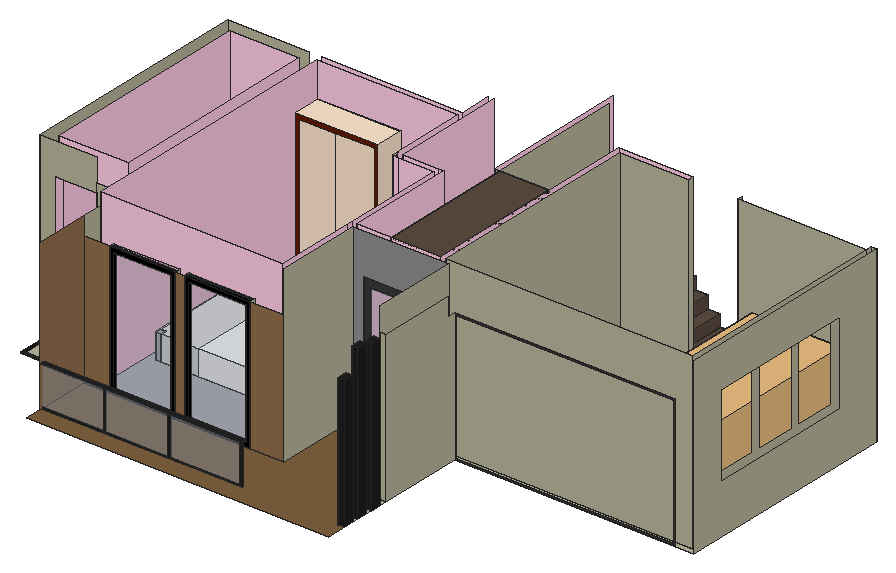
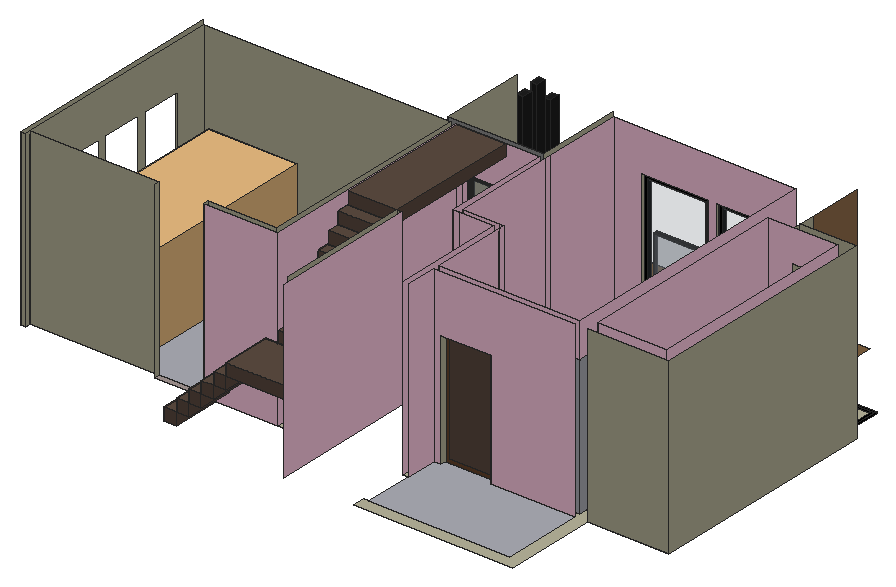
# SketchUp Ruby script. Lengths in inches.
U = 1.inch
M = Sketchup.active_model
def pt(a) = Geom::Point3d.new(a.map { |v| v * U })
def face(e, loops, mat)
  f = e.add_face(loops[0].map { |a| pt(a) })
  loops[1..].each { |l| e.add_face(l.map { |a| pt(a) }).erase! }
  f.material = f.back_material = mat if mat
  f
end
# faces: each face lists its corners as indices into pts; further lists are holes
def faces(e, pts, list, mat = nil) = list.each { |f| face(e, (f[0].is_a?(Array) ? f : [f]).map { |l| l.map { |i| pts[i] } }, mat) }
# xy, xz, yz: faces in a plane at the given z, y or x. An outline is a flat list of corners, or four numbers for a rectangle; further outlines are holes
def ring(l) = l.size == 4 ? [[l[0], l[1]], [l[2], l[1]], [l[2], l[3]], [l[0], l[3]]] : l.each_slice(2).to_a
def flat(e, list, mat, &to3) = list.each { |f| face(e, (f[0].is_a?(Array) ? f : [f]).map { |l| ring(l).map { |u, v| to3.(u, v) } }, mat) }
def xy(e, z, list, mat = nil) = flat(e, list, mat) { |x, y| [x, y, z] }
def xz(e, y, list, mat = nil) = flat(e, list, mat) { |x, z| [x, y, z] }
def yz(e, x, list, mat = nil) = flat(e, list, mat) { |y, z| [x, y, z] }
def lines(e, pts, list) = list.each { |a, b| e.add_line(pt(pts[a]), pt(pts[b])) }
# prism: a flat outline (further loops are holes) pulled along v
def prism(e, loops, v, mat = nil)
  f = face(e, loops, mat); d = Geom::Vector3d.new(v.map { |x| x * U })
  f.pushpull(f.normal.samedirection?(d) ? d.length : -d.length)
end
def box(e, o, s, mat = nil) = prism(e, [[o, [o[0] + s[0], o[1], o[2]], [o[0] + s[0], o[1] + s[1], o[2]], [o[0], o[1] + s[1], o[2]]]], [0, 0, s[2]], mat)
def at(x, y, z, deg = 0) = Geom::Transformation.translation(pt([x, y, z])) * Geom::Transformation.rotation(ORIGIN, Z_AXIS, deg.degrees)
def axes(o, x, y, z) = Geom::Transformation.new([*x, 0, *y, 0, *z, 0, *pt(o).to_a, 1])
def part(name) = M.definitions.add(name)
# library, detail: a bought-in or finely detailed component or shape, given as its bounding box
def library(name, o, s) = part(name).tap { |d| box(d.entities, o, s) }
def detail(e, o, s) = box(e.add_group.entities, o, s)
def put(e, d, t, mat = nil) = e.add_instance(d, t).tap { |i| i.material = mat if mat }
def group(e, t, mat = nil) = e.add_group.tap { |g| g.transformation = t; g.material = mat if mat }.entities
root = M.entities
M.materials.add("B08_Burnt_Sienna").color = [102, 25, 0]
M.materials.add("C01_Vanilla_Cream").color = [255, 230, 206]
M.materials.add("Concrete_04_1K").color = [184, 181, 156]
M.materials.add("Glass_Basic_01").color = [161, 173, 186]
M.materials["Glass_Basic_01"].alpha = 0.25
M.materials.add("L01_Cotton_Candy").color = [255, 204, 229]
M.materials.add("M00_Soft_Cloud").color = [255, 255, 255]
M.materials.add("M01_Silver_Fog").color = [224, 224, 224]
M.materials.add("M04_Stone_Frost").color = [142, 142, 142]
M.materials.add("M07_Charcoal_Gleam").color = [58, 58, 58]
M.materials.add("M08_Obsidian_Black").color = [30, 30, 30]
M.materials.add("M09_Shadow_Night").color = [0, 0, 0]
M.materials.add("Marble_03_1K").color = [175, 182, 201]
M.materials.add("Marble_06_1K").color = [165, 150, 147]
M.materials.add("Marble_20_1K").color = [172, 173, 182]
M.materials.add("Plywood_01_1K").color = [125, 96, 64]
M.materials.add("Wood_Floor_01_1K").color = [146, 111, 76]
M.materials.add("Wood_Floor_12_1K1").color = [92, 75, 65]
M.materials.add("Wood_Veneer_15_1K").color = [103, 69, 45]
c1 = part("Group\#4")
xy(c1.entities,0,[[0,-2.09,48,0]],"M09_Shadow_Night")
xy(c1.entities,3,[[3,-2.09,45,0]],"M09_Shadow_Night")
xy(c1.entities,93,[[3,-2.09,45,0]],"M09_Shadow_Night")
xy(c1.entities,96,[[0,-2.09,48,0]],"M09_Shadow_Night")
xz(c1.entities,-2.09,[[[0,0,48,96],[3,3,45,93]]],"M09_Shadow_Night")
xz(c1.entities,0,[[3,3,45,93]],"Glass_Basic_01")
xz(c1.entities,0,[[[0,0,48,96],[3,3,45,93]]],"M09_Shadow_Night")
yz(c1.entities,0,[[-2.09,0,0,96]],"M09_Shadow_Night")
yz(c1.entities,3,[[-2.09,3,0,93]],"M09_Shadow_Night")
yz(c1.entities,45,[[-2.09,3,0,93]],"M09_Shadow_Night")
yz(c1.entities,48,[[-2.09,0,0,96]],"M09_Shadow_Night")
c2 = library("Car 018",[-39.37,-94.12,-0.14],[78.74,183.68,64.54])
c3 = part("Group\#29")
box(c3.entities,[0,0,0],[9,36,9])
xy(root,15,[[4695.7,3573.98,4700.3125,3604.45],[4480,3604.45,4480,3639.11,4462.07,3639.11,4462.07,3645.11,4480,3645.11,4480,3800.79,4429.38,3800.79,4429.38,3645.11,4432.07,3645.11,4432.07,3639.11,4420.38,3639.11,4420.38,3809.79,4480,3809.79,4480,3878.04,4595.8125,3878.04,4595.8125,3869.04,4489,3869.04,4489,3809.79,4550.5625,3809.79,4550.5625,3805.79,4489,3805.79,4489,3608.64,4498.625,3608.64,4498.625,3604.45],[4546.625,3604.45,4553.37,3608.64],[4601.37,3604.45,4601.37,3608.64,4621.87,3608.64,4621.87,3746.01,4591.8125,3746.01,4591.8125,3805.79,4586.5625,3805.79,4586.5625,3809.79,4591.8125,3809.79,4591.8125,3833.04,4595.8125,3833.04,4595.8125,3750.01,4625.87,3750.01,4625.87,3670.98,4634.06,3670.98,4634.06,3666.98,4625.87,3666.98,4625.87,3604.45],[4695.7,3604.45,4700.3125,3666.98],
  [4498.625,3606.54,4546.625,3608.64],[4432.07,3611.04,4462.07,3645.11],[4462.07,3611.04,4472.4375,3639.11],[4634.06,3666.98,4682.06,3670.98],[4682.06,3666.98,4682.06,3670.98,4686.8125,3670.98,4686.8125,3833.04,4690.8125,3833.04,4690.8125,3670.98,4870.8125,3670.98,4870.8125,3833.04,4874.8125,3833.04,4874.8125,3666.98],
  [4650.8125,3770.04,4686.8125,3779.04],[4650.8125,3779.04,4686.8125,3788.04],[4650.8125,3788.04,4686.8125,3797.04],[4650.8125,3797.04,4686.8125,3806.04],[4650.8125,3806.04,4686.8125,3815.04],
  [4650.8125,3815.04,4686.8125,3824.04],[4650.8125,3824.04,4686.8125,3833.04]],"Concrete_04_1K")
xy(root,15,[[4430.07,3609.04,4430.07,3639.11,4432.07,3639.11,4432.07,3611.04,4472.4375,3611.04,4472.4375,3609.04]],"M09_Shadow_Night")
xy(root,15,[[4429.38,3645.11,4480,3800.79]],"Marble_03_1K")
xy(root,15,[[4625.87,3670.98,4686.8125,3750.01],[4741.125,3829.04,4777.125,3833.04]],"Marble_06_1K")
xy(root,15,[[4489,3608.64,4621.87,3608.64,4621.87,3746.01,4591.8125,3746.01,4591.8125,3805.79,4549.875,3805.79,4549.875,3785.04,4489,3785.04],[4690.8125,3670.98,4870.8125,3829.04],[4550.5625,3805.79,4586.5625,3805.79,4586.5625,3809.79,4591.8125,3809.79,4591.8125,3869.04,4489,3869.04,4489,3809.79,4550.5625,3809.79]],"Marble_20_1K")
xy(root,15,[[4480,3552.7,4700.3125,3552.7,4700.3125,3566.51,4695.7,3566.51,4695.7,3666.98,4625.87,3666.98,4625.87,3604.45,4601.37,3604.45,4601.37,3608.64,4553.37,3608.64,4553.37,3604.45,4546.625,3604.45,4546.625,3606.54,4498.625,3606.54,4498.625,3604.45,4480,3604.45]],"Plywood_01_1K")
xz(root,3604.45,[[4695.7,15,4700.3125,124.125]],"Concrete_04_1K")
xz(root,3604.45,[[4480,15,4498.625,111],[4546.625,15,4553.37,111],[4601.37,15,4625.87,111]],"Wood_Floor_01_1K")
xz(root,3608.64,[[4489,15,4489,141,4621.87,141,4621.87,15,4601.37,15,4601.37,111,4553.37,111,4553.37,15,4546.625,15,4546.625,111,4498.625,111,4498.625,15]],"L01_Cotton_Candy")
xz(root,3609.04,[[4462.07,15,4472.4375,16]],"Concrete_04_1K")
xz(root,3609.04,[[4430.07,15,4462.07,16]],"M09_Shadow_Night")
xz(root,3611.04,[[4462.07,15,4472.4375,16]],"Concrete_04_1K")
xz(root,3611.04,[[4432.07,15,4462.07,16]],"M09_Shadow_Night")
xz(root,3639.11,[[4420.38,15,4430.07,15,4430.07,16,4430.76,16,4430.76,40,4430.07,40,4430.07,41.8125,4432.07,41.8125,4432.07,117.5625,4462.07,117.5625,4462.07,141,4420.38,141],[4462.07,15,4480,124.125]],"Concrete_04_1K")
xz(root,3639.11,[[4430.07,15,4432.07,16]],"M09_Shadow_Night")
xz(root,3645.11,[[4429.38,15,4429.38,141,4480,141,4480,15,4462.07,15,4462.07,117.5625,4432.07,117.5625,4432.07,15]],"L01_Cotton_Candy")
xz(root,3666.98,[[4625.87,15,4634.06,15,4634.06,111,4682.06,111,4682.06,15,4695.7,15,4695.7,141,4625.87,141]],"M04_Stone_Frost")
xz(root,3666.98,[[[4700.3125,15,4861.07,111],[4701.3125,16,4860.07,110]]],"M07_Charcoal_Gleam")
xz(root,3670.98,[[4690.8125,15,4870.8125,141]],"Concrete_04_1K")
xz(root,3670.98,[[4625.87,15,4625.87,141,4686.8125,141,4686.8125,15,4682.06,15,4682.06,111,4634.06,111,4634.06,15]],"L01_Cotton_Candy")
xz(root,3746.01,[[4591.8125,15,4595.8125,141],[4595.8125,15,4621.87,141]],"L01_Cotton_Candy")
xz(root,3750.01,[[4595.8125,15,4621.87,141],[4621.87,15,4625.87,141]],"L01_Cotton_Candy")
xz(root,3770.04,[[4646.8125,15,4650.8125,141]],"Concrete_04_1K")
xz(root,3800.79,[[4429.38,15,4480,141]],"L01_Cotton_Candy")
xz(root,3805.79,[[4489,15,4550.5625,15,4550.5625,99,4586.5625,99,4586.5625,15,4591.8125,15,4591.8125,141,4489,141]],"L01_Cotton_Candy")
xz(root,3809.79,[[4420.38,15,4480,141]],"Concrete_04_1K")
xz(root,3809.79,[[4489,15,4489,141,4591.8125,141,4591.8125,15,4586.5625,15,4586.5625,99,4550.5625,99,4550.5625,15]],"L01_Cotton_Candy")
xz(root,3829.04,[[4690.8125,15,4741.125,141],[4777.125,15,4870.8125,141]],"Concrete_04_1K")
xz(root,3833.04,[[4870.8125,15,4874.8125,141]],"Concrete_04_1K")
xz(root,3833.04,[[4686.8125,15,4741.125,141]],"L01_Cotton_Candy")
yz(root,4420.38,[[3639.11,15,3809.79,141]],"Concrete_04_1K")
yz(root,4429.38,[[3645.11,15,3800.79,141]],"L01_Cotton_Candy")
yz(root,4430.07,[[3609.04,15,3639.11,16]],"M09_Shadow_Night")
yz(root,4432.07,[[3639.11,15,3645.11,117.5625]],"L01_Cotton_Candy")
yz(root,4432.07,[[3611.04,15,3639.11,16]],"M09_Shadow_Night")
yz(root,4462.07,[[3639.11,15,3645.11,117.5625]],"Concrete_04_1K")
yz(root,4472.4375,[[3609.04,15,3611.04,16]],"M09_Shadow_Night")
yz(root,4480,[[3604.45,15,3639.11,124.125]],"Concrete_04_1K")
yz(root,4480,[[3645.11,15,3800.79,141]],"L01_Cotton_Candy")
yz(root,4480,[[3564.51,15,3604.45,124.125]],"Wood_Floor_01_1K")
yz(root,4489,[[3608.64,15,3805.79,141]],"L01_Cotton_Candy")
yz(root,4498.625,[[3604.45,15,3606.54,111],[3606.54,15,3608.64,111]],"Concrete_04_1K")
yz(root,4546.625,[[3604.45,15,3606.54,111],[3606.54,15,3608.64,111]],"Concrete_04_1K")
yz(root,4550.5625,[[3805.79,15,3809.79,99]],"Concrete_04_1K")
yz(root,4553.37,[[3604.45,15,3608.64,111]],"Concrete_04_1K")
yz(root,4586.5625,[[3805.79,15,3809.79,99]],"Concrete_04_1K")
yz(root,4591.8125,[[3746.01,15,3750.01,141],[3750.01,15,3750.54,141],[3750.54,15,3805.79,141],[3809.79,15,3833.04,141]],"L01_Cotton_Candy")
yz(root,4595.8125,[[3750.01,15,3833.04,141]],"L01_Cotton_Candy")
yz(root,4601.37,[[3604.45,15,3608.64,111]],"Concrete_04_1K")
yz(root,4621.87,[[3608.64,15,3666.98,141],[3666.98,15,3670.98,141],[3670.98,15,3746.01,141]],"L01_Cotton_Candy")
yz(root,4625.87,[[3604.45,15,3666.98,141]],"Concrete_04_1K")
yz(root,4625.87,[[3670.98,15,3750.01,141]],"L01_Cotton_Candy")
yz(root,4634.06,[[3666.98,15,3670.98,111]],"L01_Cotton_Candy")
yz(root,4646.8125,[[3770.04,15,3878.04,141]],"L01_Cotton_Candy")
yz(root,4650.8125,[[3770.04,15,3869.04,141]],"Concrete_04_1K")
yz(root,4682.06,[[3666.98,15,3670.98,111]],"L01_Cotton_Candy")
yz(root,4686.8125,[[3670.98,15,3833.04,141]],"L01_Cotton_Candy")
yz(root,4690.8125,[[3670.98,15,3829.04,141]],"Concrete_04_1K")
yz(root,4695.7,[[3604.45,15,3666.98,141]],"Concrete_04_1K")
yz(root,4700.3125,[[3604.45,15,3666.98,15,3666.98,111,3660.98,111,3660.98,124.125,3604.45,124.125]],"Concrete_04_1K")
yz(root,4741.125,[[3829.04,15,3833.04,141]],"Concrete_04_1K")
yz(root,4777.125,[[3829.04,15,3833.04,141]],"Concrete_04_1K")
yz(root,4870.8125,[[[3670.98,15,3829.04,141],[3694.73,54,3724.73,108],[3730.73,54,3760.73,108],[3766.73,54,3796.73,108]],[3829.04,15,3833.04,141]],"Concrete_04_1K")
yz(root,4874.8125,[[[3666.98,15,3833.04,141],[3691.73,51,3799.73,111]]],"Concrete_04_1K")
g1 = group(root,at(4480,3566.51,15))
xy(g1,0,[[0,0,145.87,0.86]])
xy(g1,30,[[0,0,145.87,0.86]])
xy(g1,30,[[0,-2,145.87,0]],"M08_Obsidian_Black")
xy(g1,31,[[0,-2,145.87,0.86]],"M08_Obsidian_Black")
xz(g1,-2,[[0,30,145.87,31]],"M08_Obsidian_Black")
xz(g1,0,[[0,1,44.62,30],[46.62,1,91.93,30],[93.93,1,143.87,30]],"Glass_Basic_01")
xz(g1,0,[[0,0,44.62,1],[44.62,0,46.62,1],[46.62,0,91.93,1],[91.93,0,93.93,1],[93.93,0,143.87,1],
  [143.87,0,145.87,30],[44.62,1,46.62,30],[91.93,1,93.93,30]],"M08_Obsidian_Black")
xz(g1,0.86,[[0,0,145.87,30]],"Glass_Basic_01")
xz(g1,0.86,[[0,30,145.87,31]],"M08_Obsidian_Black")
yz(g1,0,[[0,0,0.86,30],[-2,30,0.86,31]])
yz(g1,145.87,[[0,0,0.86,30],[-2,30,0.86,31]],"M08_Obsidian_Black")
g2 = group(root,at(4695.7,3566.51,15),"M08_Obsidian_Black")
box(g2,[0,0,0],[4.61,7.46,96])
g3 = group(root,at(4695.7,3578.89,15),"M08_Obsidian_Black")
box(g3,[0,0,0],[4.61,7.46,111.61])
g4 = group(root,at(4695.7,3591.33,15),"M08_Obsidian_Black")
box(g4,[0,0,0],[4.61,7.46,109.0625])
put(root,c1,at(4498.625,3606.54,15))
put(root,c1,at(4553.37,3606.54,15))
g5 = group(root,at(4634.06,3666.98,15))
xz(g5,0,[[5,5,43,91]],"Glass_Basic_01")
xz(g5,0,[[[0,0,48,96],[5,5,43,91]]],"M07_Charcoal_Gleam")
g6 = group(root,at(4494.8,3651.57,15))
xy(g6,0,[[4,0,4,4,0,4,0,64.6875,4.3125,64.6875,4.3125,68.6875,95.5,68.6875,95.5,64.6875,99.5,64.6875,99.5,4,95.5,4,95.5,0]])
xy(g6,18.0625,[[31.6,0,95.5,0,95.5,4,99.5,4,99.5,64.6875,95.5,64.6875,95.5,68.6875,31.6,68.6875]],"M00_Soft_Cloud")
xy(g6,18.0625,[[4,0,31.6,0,31.6,68.6875,4.3125,68.6875,4.3125,64.6875,0,64.6875,0,4,4,4]],"M01_Silver_Fog")
xy(g6,18.0625,[[0,0,4,4],[95.5,0,99.5,4],[0,64.6875,4.3125,68.6875],[95.5,64.6875,99.5,68.6875]],"Marble_20_1K")
xz(g6,0,[[31.6,0,95.5,18.0625]],"M00_Soft_Cloud")
xz(g6,0,[[4,0,31.6,18.0625]],"M01_Silver_Fog")
xz(g6,0,[[0,0,4,18.0625],[95.5,0,99.5,18.0625]],"Marble_20_1K")
xz(g6,4,[[0,0,4,18.0625],[95.5,0,99.5,18.0625]],"Marble_20_1K")
xz(g6,64.6875,[[0,0,4.3125,18.0625],[95.5,0,99.5,18.0625]],"Marble_20_1K")
xz(g6,68.6875,[[31.6,0,95.5,18.0625]],"M00_Soft_Cloud")
xz(g6,68.6875,[[4.3125,0,31.6,18.0625]],"M01_Silver_Fog")
xz(g6,68.6875,[[0,0,4.3125,18.0625],[95.5,0,99.5,18.0625]],"Marble_20_1K")
yz(g6,0,[[4,0,64.6875,18.0625]],"C01_Vanilla_Cream")
yz(g6,0,[[0,0,4,18.0625],[64.6875,0,68.6875,18.0625]],"Marble_20_1K")
yz(g6,4,[[0,0,4,18.0625]],"Marble_20_1K")
yz(g6,4.3125,[[64.6875,0,68.6875,18.0625]],"Marble_20_1K")
yz(g6,95.5,[[0,0,4,18.0625],[64.6875,0,68.6875,18.0625]],"Marble_20_1K")
yz(g6,99.5,[[4,0,64.6875,18.0625]],"M01_Silver_Fog")
yz(g6,99.5,[[0,0,4,18.0625],[64.6875,0,68.6875,18.0625]],"Marble_20_1K")
put(root,c2,axes([4829.53,3749.11,15],[0.82,0,0],[0,0.7565,0],[0,0,1]))
g7 = group(root,at(4650.8125,3670.98,15),"Wood_Floor_12_1K1")
put(g7,c3,at(0,162.0625,54,-90))
put(g7,c3,at(0,108.0625,108,-90))
put(g7,c3,at(0,135.0625,81,-90))
put(g7,c3,at(0,117.0625,99,-90))
put(g7,c3,at(0,153.0625,63,-90))
g8 = group(g7,at(0,99.0625,117,-90))
box(g8,[0,0,0],[99.0625,36,9])
put(g7,c3,at(0,126.0625,90,-90))
put(g7,c3,at(0,144.0625,72,-90))
put(g7,c3,at(72.3125,162.0625,9))
g9 = group(g7,at(63.3125,162.0625,18))
box(g9,[0,0,0],[9,36,9])
put(g7,c3,at(81.3125,162.0625,0))
g10 = group(g7,at(36.3125,162.0625,45))
box(g10,[-36.3125,0,0],[45.3125,36,9])
put(g7,c3,at(45.3125,162.0625,36))
put(g7,c3,at(54.3125,162.0625,27))
g11 = group(root,at(4489,3785.04,15))
xy(g11,0,[[0,0,60.875,20.75]],"Marble_20_1K")
xy(g11,100.625,[[0,0,60.875,20.75]],"C01_Vanilla_Cream")
xz(g11,0,[[[0,0,60.875,100.625],[3,3,57.875,97.625]]],"B08_Burnt_Sienna")
xz(g11,0,[[3,3,30.4375,97.625],[30.4375,3,57.875,97.625]],"C01_Vanilla_Cream")
xz(g11,20.75,[[0,0,60.875,100.625]],"Marble_20_1K")
yz(g11,0,[[0,0,20.75,100.625]],"Marble_20_1K")
yz(g11,60.875,[[0,0,20.75,100.625]],"C01_Vanilla_Cream")
g12 = group(root,at(4550.5625,3805.79,15))
xz(g12,0,[[3,3,33,81]],"Wood_Floor_12_1K1")
xz(g12,0,[[[0,0,36,84],[3,3,33,81]]],"Wood_Veneer_15_1K")
